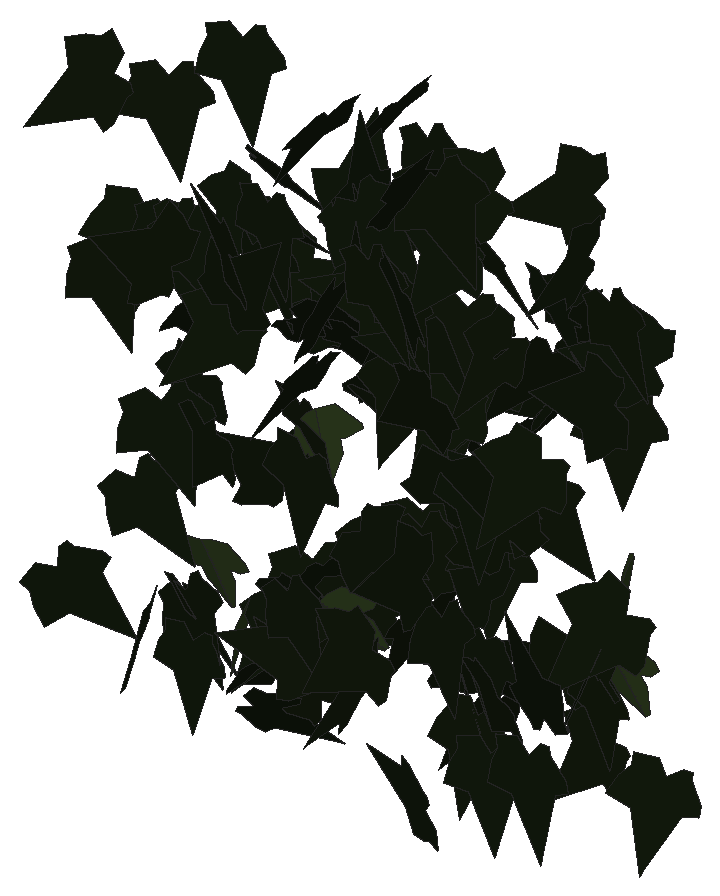
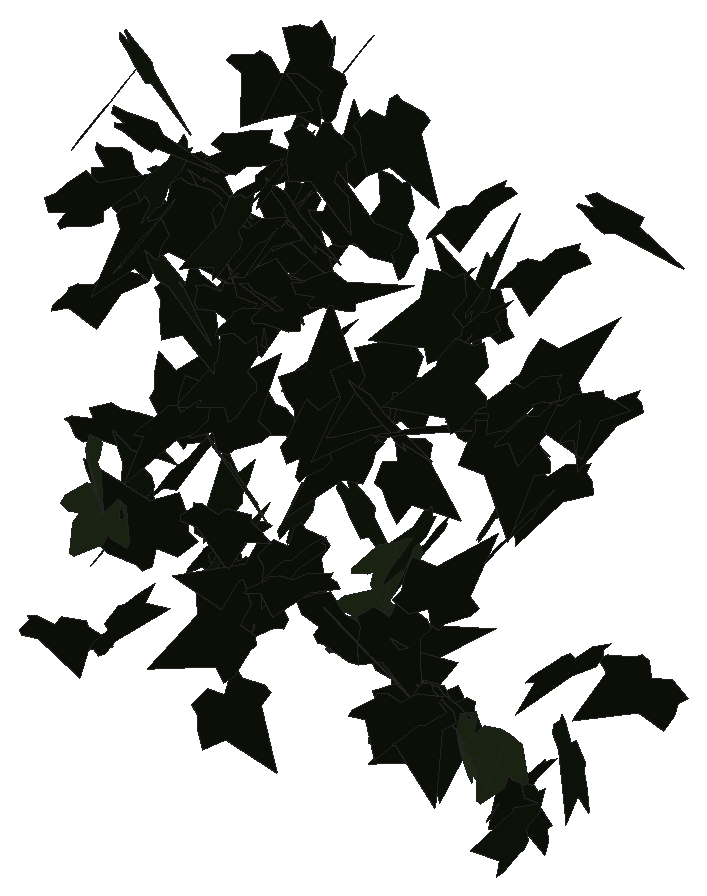
# SketchUp Ruby script. Lengths in inches.
U = 1.inch
M = Sketchup.active_model
def pt(a) = Geom::Point3d.new(a.map { |v| v * U })
def face(e, loops, mat)
  f = e.add_face(loops[0].map { |a| pt(a) })
  loops[1..].each { |l| e.add_face(l.map { |a| pt(a) }).erase! }
  f.material = f.back_material = mat if mat
  f
end
# faces: each face lists its corners as indices into pts; further lists are holes
def faces(e, pts, list, mat = nil) = list.each { |f| face(e, (f[0].is_a?(Array) ? f : [f]).map { |l| l.map { |i| pts[i] } }, mat) }
# xy, xz, yz: faces in a plane at the given z, y or x. An outline is a flat list of corners, or four numbers for a rectangle; further outlines are holes
def ring(l) = l.size == 4 ? [[l[0], l[1]], [l[2], l[1]], [l[2], l[3]], [l[0], l[3]]] : l.each_slice(2).to_a
def flat(e, list, mat, &to3) = list.each { |f| face(e, (f[0].is_a?(Array) ? f : [f]).map { |l| ring(l).map { |u, v| to3.(u, v) } }, mat) }
def xy(e, z, list, mat = nil) = flat(e, list, mat) { |x, y| [x, y, z] }
def xz(e, y, list, mat = nil) = flat(e, list, mat) { |x, z| [x, y, z] }
def yz(e, x, list, mat = nil) = flat(e, list, mat) { |y, z| [x, y, z] }
def lines(e, pts, list) = list.each { |a, b| e.add_line(pt(pts[a]), pt(pts[b])) }
# prism: a flat outline (further loops are holes) pulled along v
def prism(e, loops, v, mat = nil)
  f = face(e, loops, mat); d = Geom::Vector3d.new(v.map { |x| x * U })
  f.pushpull(f.normal.samedirection?(d) ? d.length : -d.length)
end
def box(e, o, s, mat = nil) = prism(e, [[o, [o[0] + s[0], o[1], o[2]], [o[0] + s[0], o[1] + s[1], o[2]], [o[0], o[1] + s[1], o[2]]]], [0, 0, s[2]], mat)
def at(x, y, z, deg = 0) = Geom::Transformation.translation(pt([x, y, z])) * Geom::Transformation.rotation(ORIGIN, Z_AXIS, deg.degrees)
def axes(o, x, y, z) = Geom::Transformation.new([*x, 0, *y, 0, *z, 0, *pt(o).to_a, 1])
def part(name) = M.definitions.add(name)
# library, detail: a bought-in or finely detailed component or shape, given as its bounding box
def library(name, o, s) = part(name).tap { |d| box(d.entities, o, s) }
def detail(e, o, s) = box(e.add_group.entities, o, s)
def put(e, d, t, mat = nil) = e.add_instance(d, t).tap { |i| i.material = mat if mat }
def group(e, t, mat = nil) = e.add_group.tap { |g| g.transformation = t; g.material = mat if mat }.entities
root = M.entities
M.materials.add("efeu1").color = [18, 25, 13]
M.materials.add("efeu2").color = [43, 57, 29]
c1 = part("ivyleaf_9")
p = [[1.54,2.16,1.25],[1.36,2.04,1.19],[-0.21,0.99,0.68],[-0.71,1.11,0.82],[-0.85,0.86,0.67],[-0.8,0.17,0.21],
  [-0.9,-0.01,0.1],[-0.67,-0.16,-0.02],[-0.08,-0.08,-0.05],[-0.03,-0.6,-0.4],[0.65,-0.88,-0.66],[0.83,-0.6,-0.49],
  [1.29,-0.42,-0.43],[1.8125,-0.07,-0.26],[1.21,0.44,0.15]]
faces(c1.entities,p,[[0,1,2,3,4,5,6,7,8,9,10,11,12,13,14]],"efeu1")
c2 = part("ivyleaf_10")
p = [[0,0.5,-0.03],[-0.0625,2.02,-0.43],[-0.19,2.01,-0.46],[-0.54,1.05,-0.29],[-0.52,0.625,-0.18],[-0.83,0.76,-0.28],
  [-1.16,0.64,-0.33],[-1.15,0.33,-0.24],[-0.77,-0.39,0.02],[-0.3,-0.51,0.16],[0.04,-0.48,0.23],[-0.02,2.01,-0.4375],
  [-0.06,2.01,-0.43],[0.04,-0.49,0.23],[0.67,-0.49,0.14],[1.38,0.36,-0.2],[1.375,0.51,-0.24],[0.81,0.65,-0.19],
  [0.62,0.59,-0.15],[0.6,1.09,-0.28],[0.5,1.23,-0.31]]
faces(c2.entities,p,[[0,1,2,3,4,5,6,7,8,9,10],[11,12,0,13,14,15,16,17,18,19,20]],"efeu2")
put(root,c1,axes([625.1875,111,316.64],[-0.20334,-0.39754,1.37191],[-0.60968,-1.229,-0.44649],[1.29169,-0.64268,0.00522]))
put(root,c1,axes([622.39,111.4,312.29],[-0.704,-0.78621,1.05007],[-0.12625,-1.14559,-0.94237],[1.30569,-0.53467,0.47505]))
put(root,c1,axes([625.16,111.2,306.46],[0.56078,-1.30141,0.24463],[-0.07833,0.2326,1.41695],[-1.32188,-0.56587,0.01981]))
put(root,c1,axes([621.57,112.53,328.44],[0.68943,-1.28051,-0.16061],[-0.05825,0.15103,-1.45418],[1.28923,0.6916,0.02019]))
put(root,c1,axes([622.46,113.31,327.18],[0.36522,-0.8913,1.08843],[0.35112,-1.03117,-0.96222],[1.36228,0.50473,-0.04379]))
put(root,c1,axes([628.75,113.25,308.95],[0.24745,-1.41829,0.05295],[0.01151,-0.05175,-1.43971],[1.41923,0.24771,0.00244]))
put(root,c1,axes([629.01,113.48,321.95],[-1.06341,-0.86123,0.10606],[-0.0784,-0.07171,-1.3684],[0.86419,-1.06627,0.00637]))
put(root,c1,axes([620.9,112.8,309.85],[-1.17356,0.87514,-0.27672],[0.22533,-0.16072,-1.46393],[-0.88976,-1.19498,-0.00576]))
put(root,c1,axes([624.11,113.7,313.18],[-0.57307,-0.43894,-1.08951],[1.09749,0.23193,-0.6707],[0.4186,-1.20899,0.26689]))
put(root,c1,axes([624.79,113.18,318.98],[-0.27347,-0.1721,1.42562],[1.42951,-0.17012,0.25368],[0.13605,1.4416,0.20012]))
put(root,c1,axes([629.07,113.65,310.92],[0.62195,-0.51307,1.18328],[-0.70736,0.96277,0.78926],[-1.07844,-0.92738,0.16473]))
put(root,c1,axes([625.18,114.67,319.24],[0.125,-1.4241,0.3036],[0.04971,-0.30037,-1.4294],[1.45526,0.13259,0.02275]))
put(root,c1,axes([623.41,113.84,322.66],[0.15529,0.25106,-1.28978],[-1.17613,-0.55256,-0.24916],[-0.58591,1.17573,0.15832]))
put(root,c1,axes([625.51,114.98,307.13],[-0.04194,-1.30498,-0.14788],[0.00199,0.1479,-1.30565],[1.31333,-0.04189,-0.00275]))
put(root,c1,axes([616.14,115.34,316.64],[0.10987,-1.33462,0.44618],[0.06096,-0.44261,-1.33893],[1.40591,0.12348,0.02318]))
put(root,c1,axes([617.59,113.71,323.49],[0.25686,0.43655,1.37704],[0.3756,1.33035,-0.49181],[-1.3949,0.43861,0.12114]))
put(root,c1,axes([604.65,114.71,308.17],[-0.00627,-0.34959,-1.30411],[0.71413,1.10591,-0.29989],[1.14583,-0.69116,0.17977]))
put(root,c1,axes([615.43,115.26,310.56],[0.5956,-1.14201,-0.35397],[-0.18,0.30531,-1.28787],[1.18198,0.62195,-0.01776]))
put(root,c1,axes([624.87,116.13,309.06],[-0.14803,-0.73805,1.18023],[0.42845,-1.15342,-0.66755],[1.32442,0.29064,0.34786]))
put(root,c1,axes([620.24,115.93,325.36],[0.57984,-1.22517,-0.08795],[-0.03754,0.07954,-1.35545],[1.22775,0.58105,0.00009]))
put(root,c1,axes([608.69,115.9375,316.27],[-0.1497,-1.12936,-0.80892],[0.10812,0.80166,-1.13924],[1.38496,-0.18466,0.0015]))
put(root,c1,axes([611.97,115.94,321.97],[-0.51796,0.33562,1.261],[0.96304,-0.81715,0.61307],[0.88051,1.09117,0.07126]))
put(root,c1,axes([620.74,114.73,329.9375],[0.38259,0.88871,1.07059],[0.42744,0.98156,-0.96756],[-1.32411,0.57365,-0.00301]))
put(root,c1,axes([605.73,116.38,329.52],[-1.36579,-0.0259,0.33043],[-0.33036,-0.00669,-1.36604],[0.02674,-1.40518,0.00041]))
put(root,c1,axes([611.9,116.38,323.18],[0.46756,-1.25664,0.56074],[-0.07566,0.56785,1.33566],[-1.37399,-0.4589,0.11726]))
put(root,c1,axes([623.59,116.47,307.47],[-1.03618,-0.38841,-0.73525],[0.68756,0.26051,-1.10658],[0.46768,-1.24354,-0.00217]))
put(root,c1,axes([622.42,116.84,321],[-1.12959,-0.61964,-0.2132],[0.21062,0.05904,-1.28746],[0.62053,-1.14802,0.04887]))
put(root,c1,axes([610.0625,117.4,314.78],[-0.1036,-0.86687,1.02567],[0.11042,-1.03073,-0.86],[1.33838,0.01794,0.15034]))
put(root,c1,axes([617.73,117.43,326.3],[-0.0337,-0.40846,1.28253],[-0.01409,-1.28275,-0.4089],[1.34593,-0.02366,0.02783]))
put(root,c1,axes([618.65,115.75,314.24],[0.22254,-0.38761,-1.20915],[-0.27686,1.18323,-0.43026],[1.23921,0.33396,0.12102]))
put(root,c1,axes([618.04,116.25,328.15],[0.38162,-0.96952,-0.97267],[0.04179,1.01726,-0.99756],[1.3727,0.23856,0.30078]))
put(root,c1,axes([624.7,117.02,324.22],[-1.2709,-0.07683,-0.32492],[0.33041,-0.10552,-1.26742],[0.04801,-1.30752,0.12137]))
put(root,c1,axes([615.3,117.14,306.89],[-0.5255,0.03406,1.28189],[-1.26013,-0.27044,-0.50939],[0.23763,-1.35877,0.13352]))
put(root,c1,axes([621.43,116.78,330.2],[-0.54778,-0.65832,-1.24387],[1.01115,0.74429,-0.83921],[0.97886,-1.13724,0.17081]))
put(root,c1,axes([607.65,117.54,321.35],[-0.04979,0.04257,1.41718],[-1.08741,-0.9111,-0.01084],[0.90981,-1.08663,0.06461]))
put(root,c1,axes([604.95,117.08,321.02],[0.11169,-1.19892,-0.53814],[-0.04587,0.53619,-1.20411],[1.31336,0.12068,0.00371]))
put(root,c1,axes([629.7,117.04,323.17],[-0.47474,-0.14858,-1.35587],[-1.22868,-0.57682,0.49342],[-0.59228,1.31569,0.06321]))
put(root,c1,axes([628.43,117.12,329.13],[-1.17789,0.74236,-0.13039],[0.11091,-0.06857,-1.3923],[-0.74552,-1.1831,-0.00112]))
put(root,c1,axes([615.48,116.97,305.45],[-0.02519,0.02741,1.38699],[-1.12405,0.8126,-0.03647],[-0.81302,-1.12431,0.00745]))
put(root,c1,axes([612.73,116.7,304.11],[1.11658,0.22385,0.53376],[0.52191,0.11205,-1.13878],[-0.25024,1.23251,0.00658]))
put(root,c1,axes([615.45,117.43,330.54],[-0.52814,1.0432,-0.71727],[0.14681,-0.72147,-1.15741],[-1.25745,-0.52239,0.16613]))
put(root,c1,axes([621.41,117.61,323.13],[0.43476,-1.18671,-0.32652],[-0.08569,0.31627,-1.26355],[1.22783,0.44227,0.02744]))
put(root,c1,axes([607.08,116.51,305.08],[-0.47296,0.22933,-1.41585],[-1.25086,0.66355,0.52532],[0.70183,1.33717,-0.01786]))
put(root,c1,axes([617.46,117.35,327.31],[-0.14571,-1.0684,0.82613],[0.53531,0.71717,1.02191],[-1.23993,0.43518,0.3441]))
put(root,c1,axes([621.09,118.49,326.4],[-0.53517,-1.04783,0.62057],[-0.13032,-0.62468,-1.16716],[1.21082,-0.53037,0.14867]))
put(root,c1,axes([622.01,118.42,305.79],[-0.03824,-0.23563,1.47186],[0.38574,-1.42375,-0.21791],[1.43983,0.37518,0.09747]))
put(root,c1,axes([623.5625,118.11,314.26],[0.47489,0.17671,1.32123],[-1.31943,-0.1373,0.4926],[0.18971,-1.39725,0.11869]))
put(root,c1,axes([622.36,118.54,309.5],[0.14722,-1.23578,0.57859],[0.26038,-0.54581,-1.23203],[1.33945,0.24193,0.17591]))
put(root,c1,axes([628.46,116.62,310.09],[-0.05904,0.80555,1.17536],[-0.03209,1.17531,-0.80714],[-1.42455,-0.05986,-0.03053]))
put(root,c1,axes([629,117.95,326.82],[0.64355,-1.1734,-0.1858],[-0.06699,0.17513,-1.33806],[1.18613,0.64654,0.02524]))
put(root,c1,axes([618.34,118.7,319.4],[-0.16911,-1.2391,0.56615],[-0.03945,-0.5658,-1.25012],[1.36174,-0.17028,0.03409]))
put(root,c1,axes([610.34,118.46,319.44],[-1.14857,-0.56951,0.33037],[-0.29358,-0.1516,-1.282],[0.58932,-1.18548,0.00523]))
put(root,c1,axes([629.05,118.59,312.93],[-1.31075,-0.66381,0.23282],[-0.18666,-0.14648,-1.46854],[0.67824,-1.32318,0.04578]))
put(root,c1,axes([625.79,118.19,323.43],[-0.01285,0.72202,-1.1828],[-0.26068,-1.163,-0.7071],[-1.36102,0.21594,0.1466]))
put(root,c1,axes([619.76,118.125,310.17],[-0.31647,0.92222,-0.85565],[0.29568,-0.80306,-0.97491],[-1.22278,-0.43287,-0.01429]))
put(root,c1,axes([623.54,117.33,312.36],[-0.53526,0.82685,0.88023],[-0.56261,0.68123,-0.98203],[-1.06863,-0.77281,0.07612]))
put(root,c1,axes([621.66,118.34,323.86],[-0.39231,-1.14408,-0.54111],[0.19598,0.50476,-1.20931],[1.25032,-0.43809,0.01977]))
put(root,c1,axes([620.88,118.61,320.7],[-0.3419,-1.28681,-0.31378],[0.10761,0.29601,-1.33118],[1.32013,-0.3574,0.02725]))
put(root,c1,axes([620.71,118.71,321.18],[-0.50083,-0.07317,1.26982],[-1.26316,-0.13137,-0.50577],[0.1491,-1.35868,-0.01948]))
put(root,c1,axes([607.71,118.98,304.125],[0.11044,-1.23066,0.15811],[-0.00713,-0.15936,-1.23542],[1.24076,0.10862,-0.02117]))
put(root,c2,axes([615.4,118.04,308.77],[-0.84538,-0.26673,-0.90688],[0.85937,0.28995,-0.88637],[0.39377,-1.20542,-0.01254]))
put(root,c1,axes([612.13,117.65,305.54],[0.11557,1.30987,0.14498],[0.01277,0.14441,-1.31496],[-1.3178,0.11627,-0.00003]))
put(root,c1,axes([624.78,118.38,320.1],[-0.52106,1.15113,-0.56608],[0.24445,-0.5107,-1.26352],[-1.25928,-0.57545,-0.01104]))
put(root,c1,axes([607.74,119.4,315.64],[-0.12873,-1.13554,0.68159],[0.05589,-0.68885,-1.13708],[1.32321,-0.08137,0.11434]))
put(root,c1,axes([611.42,118.99,324.62],[0.35987,-1.27124,0.13204],[0.05022,-0.123,-1.32111],[1.27709,0.36306,0.01474]))
put(root,c1,axes([617.69,118.93,322.63],[-0.70691,0.2319,1.06224],[-1.07419,-0.34484,-0.63958],[0.16809,-1.22848,0.38005]))
put(root,c1,axes([605.28,119.12,322.06],[-0.69361,-1.22984,-0.3321],[0.16526,0.28807,-1.41194],[1.26312,-0.71302,0.00236]))
put(root,c1,axes([612.16,119.0625,306.86],[-1.23025,-0.13136,-0.22513],[0.22356,0.02671,-1.23724],[0.13402,-1.2504,-0.00278]))
put(root,c1,axes([622.19,119.22,321.24],[-1.09781,-0.66312,-0.22872],[0.17357,0.15478,-1.28186],[0.67965,-1.11065,-0.04208]))
put(root,c1,axes([605.26,118.64,310.54],[0.4411,-1.0599,-0.73058],[0.08625,0.79488,-1.10111],[1.28441,0.31062,0.32484]))
put(root,c1,axes([627.21,119.4375,309.01],[0.31444,-1.17906,0.32507],[0.09213,-0.31185,-1.22024],[1.21957,0.32755,0.00837]))
put(root,c1,axes([621.6,118.75,317.72],[1.18135,-0.44659,0.29333],[0.26363,-0.13193,-1.26261],[0.46474,1.21006,-0.0294]))
put(root,c1,axes([609.86,119.81,324.03],[-0.39606,-1.12691,0.54071],[-0.07071,-0.5461,-1.18993],[1.24792,-0.38859,0.10419]))
put(root,c1,axes([624.84,119.46,325.39],[0.6525,-1.08366,0.47657],[0.25783,-0.40103,-1.26488],[1.15541,0.70147,0.01311]))
put(root,c1,axes([606.29,119.28,328.22],[-0.1872,-1.23719,-0.45577],[0.08466,0.44811,-1.25118],[1.31575,-0.20485,0.01566]))
put(root,c1,axes([620.35,118.36,307.89],[0.47462,0.09126,1.31483],[1.28373,0.28459,-0.48315],[-0.29859,1.3686,0.01279]))
put(root,c1,axes([607.3,119.1875,322.13],[0.10889,-1.09654,-0.71782],[0.05812,0.72362,-1.09659],[1.30931,0.05907,0.10838]))
put(root,c1,axes([616.7,119.5,318.49],[0.80308,0.71394,0.80886],[-0.62179,-0.51775,1.07434],[0.88167,-1.01544,0.02092]))
put(root,c1,axes([613.91,119.2,309.52],[-0.21963,1.09343,-0.60107],[0.12593,-0.58777,-1.11525],[-1.24138,-0.25308,-0.00679]))
put(root,c1,axes([621.375,120.07,328.28],[-0.96368,-0.44899,0.76497],[-0.65505,-0.40136,-1.06078],[0.59806,-1.16308,0.07075]))
put(root,c2,axes([609.74,119.8,305.9],[0.61108,-0.96069,0.51278],[0.27744,-0.43124,-1.13857],[1.05304,0.67111,0.00241]))
put(root,c1,axes([625.73,119.22,308.81],[-0.43667,0.01491,1.42325],[1.36404,-0.42083,0.42291],[0.40654,1.42802,0.10977]))
put(root,c1,axes([608.2,118.88,319.37],[0.19746,1.30743,-0.17125],[-0.03292,-0.16821,-1.32224],[-1.31819,0.20005,0.00737]))
put(root,c1,axes([625.44,119.19,321.58],[-0.92772,0.93372,0.23511],[-0.18498,0.14757,-1.31597],[-0.94493,-0.9456,0.02679]))
put(root,c1,axes([615.74,119.14,325.91],[-1.22055,0.16301,0.61936],[0.58813,-0.2424,1.22281],[0.25353,1.34706,0.1451]))
put(root,c1,axes([610.53,119.99,322.36],[0.52528,-1.19343,0.18934],[0.07859,-0.17227,-1.30391],[1.2058,0.53112,0.00251]))
put(root,c1,axes([628.97,120.38,323.17],[-0.49628,-0.03954,1.22679],[-1.05301,-0.6662,-0.44745],[0.63067,-1.14345,0.21827]))
put(root,c1,axes([616.95,119.61,308.375],[-0.64098,0.25346,1.19319],[-1.10961,0.43871,-0.68927],[-0.50666,-1.28144,0.00003]))
put(root,c1,axes([613.1875,118.78,320.41],[1.08138,0.65846,0.54013],[0.42254,0.34315,-1.26428],[-0.73944,1.15904,0.06746]))
put(root,c1,axes([605.9,119.97,321.75],[0.07119,-1.25881,-0.39591],[0.04422,0.39854,-1.25921],[1.31886,0.05458,0.06359]))
put(root,c1,axes([612.62,120.22,317.43],[-0.63061,0.58043,-0.95952],[0.36819,-0.93264,-0.80615],[-1.05925,-0.66974,0.29103]))
put(root,c1,axes([610.91,120.41,311.82],[0.25759,0.15676,1.27165],[-1.16572,-0.50967,0.29895],[0.53177,-1.19319,0.03937]))
put(root,c1,axes([626.49,120.9,305.53],[-0.386,-0.92053,0.87757],[-0.3744,-0.79421,-0.99777],[1.21545,-0.53698,-0.02866]))
put(root,c1,axes([608.99,120.42,330.33],[-0.01093,-1.35148,-0.26052],[0.01151,0.26043,-1.3515],[1.37632,-0.01291,0.00923]))
put(root,c2,axes([627.75,119.93,310.1],[-1.16215,-0.09357,-0.49205],[0.49654,-0.0521,-1.16284],[0.06572,-1.26095,0.08456]))
put(root,c1,axes([614.23,119.61,319.82],[1.32885,0.12258,-0.03253],[-0.03246,-0.00223,-1.33449],[-0.1226,1.32925,0.00076]))
put(root,c1,axes([618.67,119.64,326.375],[-0.68294,0.62888,0.92752],[-0.65993,0.65217,-0.92809],[-0.90569,-0.94941,-0.02314]))
put(root,c1,axes([618.07,120.51,329.08],[0.5138,-1.23155,-0.18048],[-0.07601,0.16385,-1.33441],[1.24238,0.51934,-0.00699]))
put(root,c1,axes([623.81,120.03,315.61],[0.34043,-0.91908,-0.92115],[-0.09713,0.93155,-0.96535],[1.29761,0.31086,0.16941]))
put(root,c1,axes([627.41,120.82,320.46],[-0.32081,-1.24261,-0.27622],[0.10222,0.25879,-1.28292],[1.26883,-0.33503,0.03352]))
put(root,c1,axes([621.3,120.7,312.24],[-0.85817,-0.68293,-0.61293],[0.48836,0.3706,-1.09668],[0.77691,-0.98732,0.01232]))
put(root,c1,axes([616.49,121.45,317.0625],[-0.01088,-0.10759,1.41416],[-0.77974,-1.18083,-0.09584],[1.18467,-0.77821,-0.05009]))
put(root,c1,axes([620.93,120.1,307.22],[1.37931,-0.12389,0.41022],[0.40854,-0.03708,-1.38486],[0.12932,1.43854,-0.00037]))
put(root,c1,axes([616.74,120.25,330.43],[-0.4077,1.19359,-0.3546],[0.0331,-0.3626,-1.25859],[-1.24471,-0.4006,0.08268]))
put(root,c1,axes([606.09,120.68,304.94],[-0.37412,-0.29937,-1.24944],[1.18743,0.41639,-0.45532],[0.49064,-1.23599,0.14924]))
put(root,c1,axes([629.14,121.05,304.74],[-0.94455,-0.75306,-0.43916],[0.36583,0.24534,-1.20752],[0.79129,-1.01235,0.03404]))
put(root,c1,axes([611.96,120.36,307.01],[0.68574,0.53888,-1.11801],[-0.94937,-0.59496,-0.86908],[-0.7994,1.16885,0.07307]))
put(root,c1,axes([617.48,120.87,311.65],[0.30377,-1.2113,-0.37192],[0.00935,0.38459,-1.24494],[1.26708,0.28756,0.09835]))
put(root,c1,axes([620.39,120.77,325.32],[1.03802,-0.82635,0.11102],[0.10095,-0.05141,-1.32659],[0.82765,1.04268,0.02257]))
put(root,c1,axes([609.88,120.6,325.26],[1.18995,-0.45056,0.42636],[0.43863,-0.04101,-1.26755],[0.43861,1.26336,0.11091]))
put(root,c1,axes([611.15,121.31,314.68],[0.5687,-1.03781,0.44412],[0.27114,-0.35715,-1.1818],[1.0958,0.62698,0.06193]))
put(root,c1,axes([614.54,121.43,310.03],[-1.19536,0.08413,-0.39144],[0.37281,-0.21554,-1.18479],[-0.146,-1.23921,0.1795]))
put(root,c2,axes([627.08,121.375,312.99],[0.6957,-1.01667,0.30384],[0.24458,-0.1999,-1.22888],[1.03253,0.73236,0.08637]))
put(root,c1,axes([625.45,120.06,323.56],[0.02814,0.16855,-1.30878],[-0.71688,1.101,0.12638],[1.10787,0.70815,0.11502]))
put(root,c1,axes([624.25,121.45,324.25],[0.52033,-1.19661,-0.04835],[-0.01541,0.04603,-1.30484],[1.19749,0.52054,0.00422]))
put(root,c1,axes([620.36,121.35,304.74],[-0.24541,0.85466,-0.86252],[0.03297,-0.87494,-0.87636],[-1.2138,-0.19656,0.15058]))
put(root,c2,axes([606.98,120.98,307.05],[-1.21754,0.04484,-0.25395],[0.25404,-0.00225,-1.21835],[-0.04436,-1.24374,-0.00695]))
put(root,c1,axes([613.46,120.77,319.72],[-0.65805,0.6636,0.93178],[-0.73332,0.5803,-0.93118],[-0.87796,-0.98209,0.07939]))
put(root,c1,axes([625.05,121.54,328.79],[-1.15751,0.25758,0.63395],[-0.64472,0.00692,-1.17999],[-0.2293,-1.31973,0.11755]))
put(root,c1,axes([608.46,121.05,322.85],[1.18624,-0.24349,0.56038],[0.56911,-0.005,-1.20689],[0.22233,1.31194,0.09941]))
put(root,c1,axes([605.32,121.61,304.3],[0.9639,-0.93429,0.32696],[0.23556,-0.22675,-1.34239],[0.96141,0.99227,0.0011]))
put(root,c1,axes([610.7,122.39,320.51],[-1.04188,-0.72682,0.36903],[0.02152,-0.62321,-1.16666],[0.81485,-0.91285,0.50266]))
put(root,c2,axes([612.02,121.32,314.16],[0.43295,1.17989,0.10803],[0.00646,0.11266,-1.25639],[-1.18481,0.43177,0.03262]))
put(root,c1,axes([611.42,121.7,307.75],[-0.32446,-1.05969,-0.76898],[0.34281,0.69585,-1.10355],[1.26363,-0.46087,0.10193]))
put(root,c1,axes([616.6,121.95,311.55],[-0.23633,-1.14024,-0.51955],[0.4206,0.42584,-1.12592],[1.18033,-0.38005,0.29719]))
